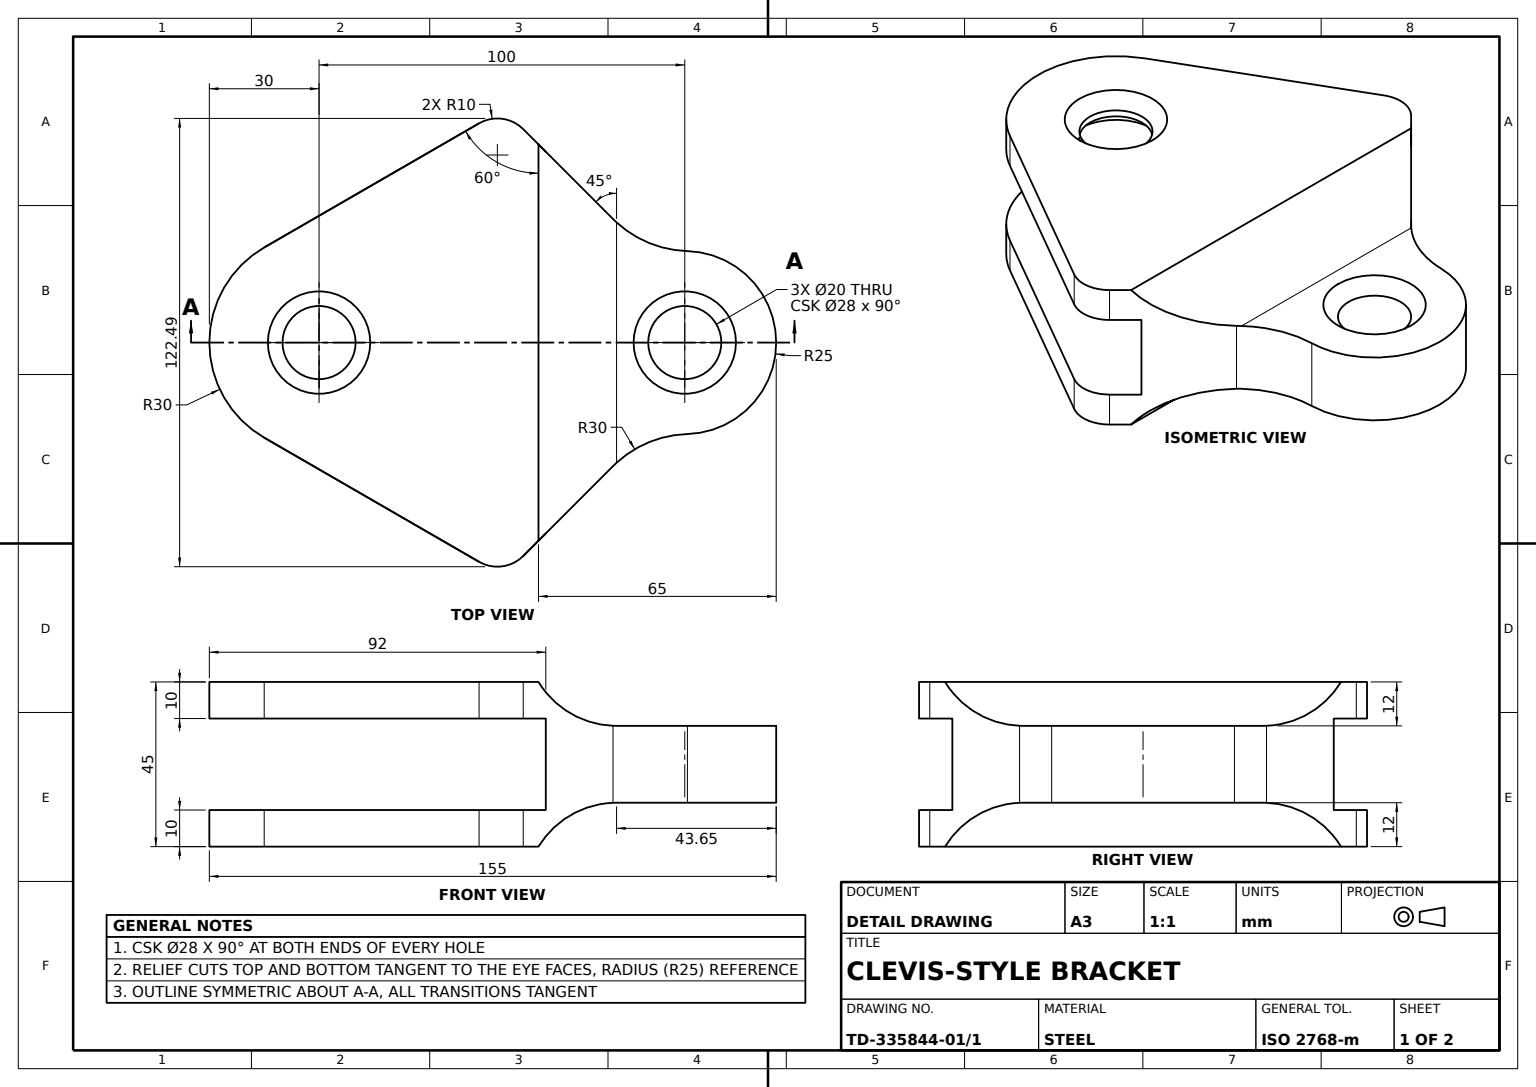
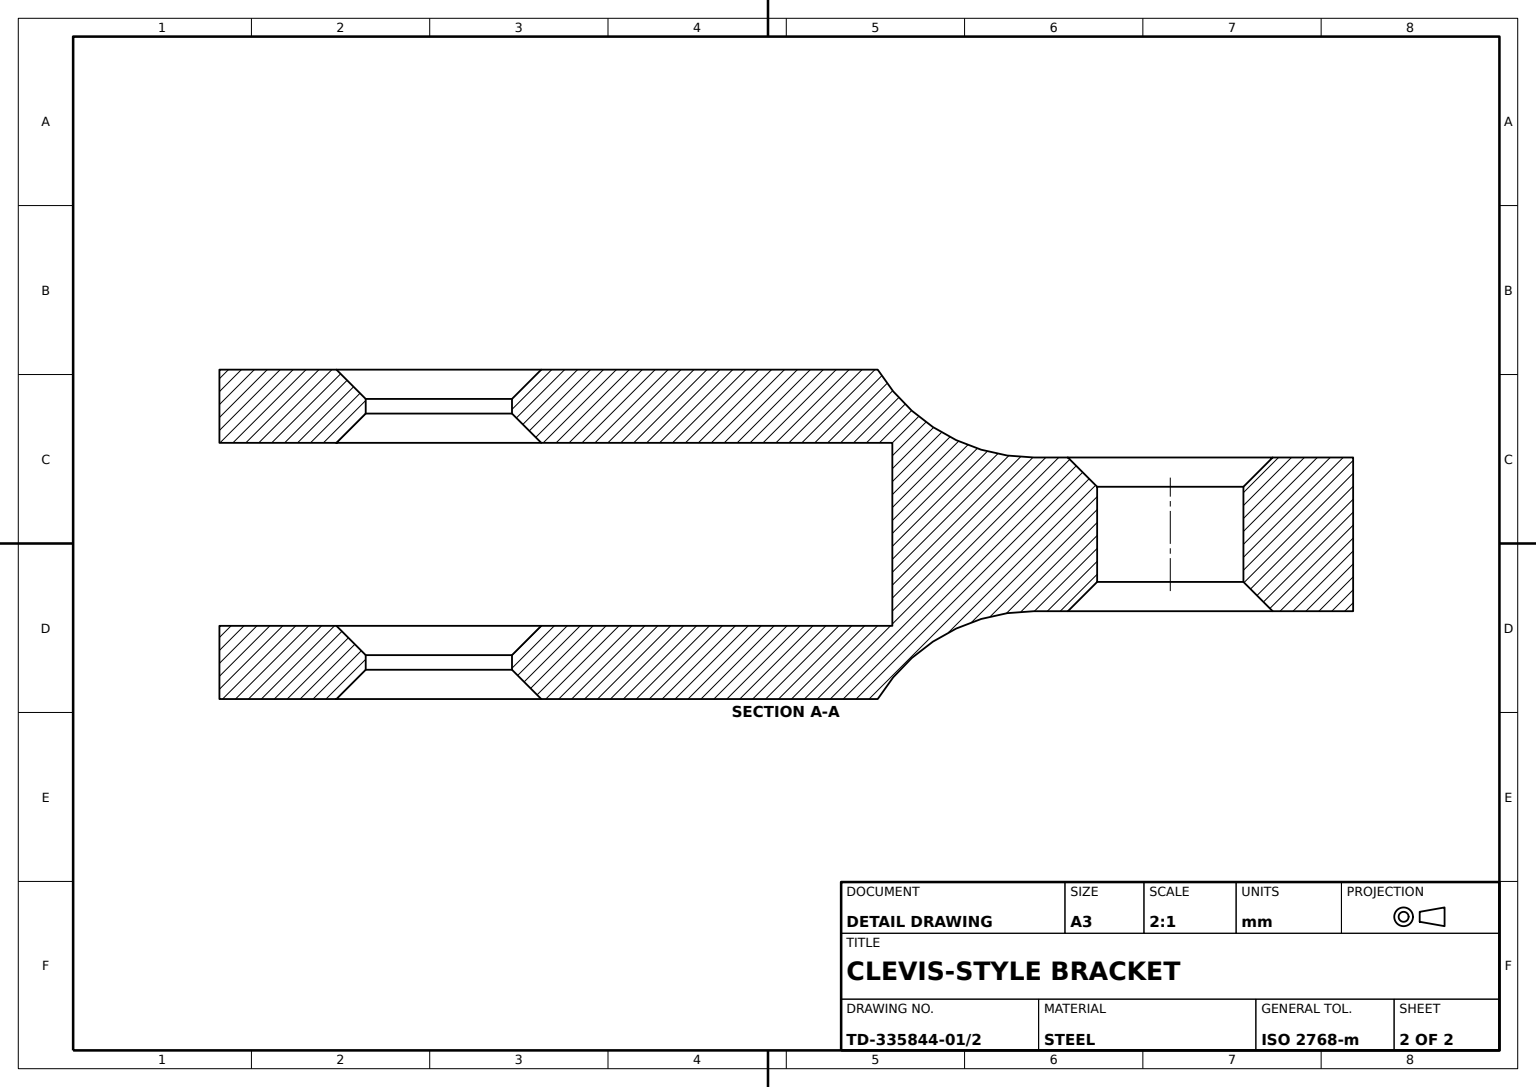
ISO-10303-21;
HEADER;
FILE_DESCRIPTION((''),'2;1');
FILE_NAME('','',(''),(''),'','','');
FILE_SCHEMA(('AUTOMOTIVE_DESIGN'));
ENDSEC;
DATA;
#1=APPLICATION_CONTEXT('');
#2=PRODUCT_CONTEXT('',#1,'mechanical');
#3=PRODUCT('','','',(#2));
#4=PRODUCT_DEFINITION_FORMATION('','',#3);
#5=PRODUCT_DEFINITION_CONTEXT('',#1,'design');
#6=PRODUCT_DEFINITION('','',#4,#5);
#7=PRODUCT_DEFINITION_SHAPE('','',#6);
#8=(LENGTH_UNIT()NAMED_UNIT(*)SI_UNIT(.MILLI.,.METRE.));
#9=(NAMED_UNIT(*)PLANE_ANGLE_UNIT()SI_UNIT($,.RADIAN.));
#10=(NAMED_UNIT(*)SI_UNIT($,.STERADIAN.)SOLID_ANGLE_UNIT());
#11=UNCERTAINTY_MEASURE_WITH_UNIT(LENGTH_MEASURE(1.E-05),#8,'distance_accuracy_value','');
#12=(GEOMETRIC_REPRESENTATION_CONTEXT(3)GLOBAL_UNCERTAINTY_ASSIGNED_CONTEXT((#11))GLOBAL_UNIT_ASSIGNED_CONTEXT((#8,#9,#10))REPRESENTATION_CONTEXT('',''));
#13=CARTESIAN_POINT('',(0.,-10.5,-86.));
#14=VERTEX_POINT('',#13);
#15=CARTESIAN_POINT('',(0.,-10.5,-114.));
#16=VERTEX_POINT('',#15);
#17=CARTESIAN_POINT('',(0.,-10.5,-100.));
#18=DIRECTION('',(0.,1.,0.));
#19=DIRECTION('',(0.,0.,1.));
#20=AXIS2_PLACEMENT_3D('',#17,#18,#19);
#21=CIRCLE('',#20,14.);
#22=EDGE_CURVE('',#14,#16,#21,.T.);
#23=ORIENTED_EDGE('',*,*,#22,.F.);
#24=CARTESIAN_POINT('',(0.,-6.5,-90.));
#25=VERTEX_POINT('',#24);
#26=DIRECTION('',(0.,-0.707106781,0.707106781));
#27=VECTOR('',#26,1000.);
#28=LINE('',#13,#27);
#29=EDGE_CURVE('',#25,#14,#28,.T.);
#30=ORIENTED_EDGE('',*,*,#29,.F.);
#31=CARTESIAN_POINT('',(0.,-6.5,-110.));
#32=VERTEX_POINT('',#31);
#33=CARTESIAN_POINT('',(0.,-6.5,-100.));
#34=DIRECTION('',(0.,-1.,0.));
#35=AXIS2_PLACEMENT_3D('',#33,#34,#19);
#36=CIRCLE('',#35,10.);
#37=EDGE_CURVE('',#32,#25,#36,.T.);
#38=ORIENTED_EDGE('',*,*,#37,.F.);
#39=DIRECTION('',(0.,-0.707106781,-0.707106781));
#40=VECTOR('',#39,1000.);
#41=LINE('',#15,#40);
#42=EDGE_CURVE('',#32,#16,#41,.T.);
#43=ORIENTED_EDGE('',*,*,#42,.T.);
#44=EDGE_LOOP('',(#23,#30,#38,#43));
#45=FACE_OUTER_BOUND('',#44,.T.);
#46=DIRECTION('',(0.,0.,-1.));
#47=AXIS2_PLACEMENT_3D('',#17,#34,#46);
#48=CONICAL_SURFACE('',#47,14.,0.785398163);
#49=ADVANCED_FACE('',(#45),#48,.F.);
#50=CARTESIAN_POINT('',(0.,16.5,-10.));
#51=VERTEX_POINT('',#50);
#52=CARTESIAN_POINT('',(0.,16.5,10.));
#53=VERTEX_POINT('',#52);
#54=CARTESIAN_POINT('',(0.,16.5,0.));
#55=AXIS2_PLACEMENT_3D('',#54,#34,#19);
#56=CIRCLE('',#55,10.);
#57=EDGE_CURVE('',#51,#53,#56,.T.);
#58=ORIENTED_EDGE('',*,*,#57,.F.);
#59=CARTESIAN_POINT('',(0.,12.5,-14.));
#60=VERTEX_POINT('',#59);
#61=LINE('',#59,#40);
#62=EDGE_CURVE('',#51,#60,#61,.T.);
#63=ORIENTED_EDGE('',*,*,#62,.T.);
#64=CARTESIAN_POINT('',(0.,12.5,14.));
#65=VERTEX_POINT('',#64);
#66=CARTESIAN_POINT('',(0.,12.5,0.));
#67=AXIS2_PLACEMENT_3D('',#66,#18,#19);
#68=CIRCLE('',#67,14.);
#69=EDGE_CURVE('',#65,#60,#68,.T.);
#70=ORIENTED_EDGE('',*,*,#69,.F.);
#71=LINE('',#64,#27);
#72=EDGE_CURVE('',#53,#65,#71,.T.);
#73=ORIENTED_EDGE('',*,*,#72,.F.);
#74=EDGE_LOOP('',(#58,#63,#70,#73));
#75=FACE_OUTER_BOUND('',#74,.T.);
#76=AXIS2_PLACEMENT_3D('',#66,#34,#46);
#77=CONICAL_SURFACE('',#76,14.,0.785398163);
#78=ADVANCED_FACE('',(#75),#77,.F.);
#79=CARTESIAN_POINT('',(25.980762,-12.5,15.));
#80=VERTEX_POINT('',#79);
#81=CARTESIAN_POINT('',(-25.980762,-12.5,15.));
#82=VERTEX_POINT('',#81);
#83=CARTESIAN_POINT('',(0.,-12.5,0.));
#84=AXIS2_PLACEMENT_3D('',#83,#34,#46);
#85=CIRCLE('',#84,30.);
#86=EDGE_CURVE('',#80,#82,#85,.T.);
#87=ORIENTED_EDGE('',*,*,#86,.T.);
#88=CARTESIAN_POINT('',(-25.980762,-22.5,15.));
#89=VERTEX_POINT('',#88);
#90=CARTESIAN_POINT('',(-25.980762,22.5,15.));
#91=VECTOR('',#34,1000.);
#92=LINE('',#90,#91);
#93=EDGE_CURVE('',#82,#89,#92,.T.);
#94=ORIENTED_EDGE('',*,*,#93,.T.);
#95=CARTESIAN_POINT('',(25.980762,-22.5,15.));
#96=VERTEX_POINT('',#95);
#97=CARTESIAN_POINT('',(0.,-22.5,0.));
#98=AXIS2_PLACEMENT_3D('',#97,#18,#19);
#99=CIRCLE('',#98,30.);
#100=EDGE_CURVE('',#89,#96,#99,.T.);
#101=ORIENTED_EDGE('',*,*,#100,.T.);
#102=CARTESIAN_POINT('',(25.980762,22.5,15.));
#103=LINE('',#102,#91);
#104=EDGE_CURVE('',#80,#96,#103,.T.);
#105=ORIENTED_EDGE('',*,*,#104,.F.);
#106=EDGE_LOOP('',(#87,#94,#101,#105));
#107=FACE_OUTER_BOUND('',#106,.T.);
#108=CARTESIAN_POINT('',(0.,22.5,0.));
#109=AXIS2_PLACEMENT_3D('',#108,#34,#46);
#110=CYLINDRICAL_SURFACE('',#109,30.);
#111=ADVANCED_FACE('',(#107),#110,.T.);
#112=CARTESIAN_POINT('',(0.,-16.5,-10.));
#113=VERTEX_POINT('',#112);
#114=CARTESIAN_POINT('',(0.,-16.5,10.));
#115=VERTEX_POINT('',#114);
#116=CARTESIAN_POINT('',(0.,-16.5,0.));
#117=AXIS2_PLACEMENT_3D('',#116,#18,#46);
#118=CIRCLE('',#117,10.);
#119=EDGE_CURVE('',#113,#115,#118,.T.);
#120=ORIENTED_EDGE('',*,*,#119,.F.);
#121=CARTESIAN_POINT('',(0.,-12.5,-14.));
#122=VERTEX_POINT('',#121);
#123=DIRECTION('',(0.,0.707106781,-0.707106781));
#124=VECTOR('',#123,1000.);
#125=LINE('',#121,#124);
#126=EDGE_CURVE('',#113,#122,#125,.T.);
#127=ORIENTED_EDGE('',*,*,#126,.T.);
#128=CARTESIAN_POINT('',(0.,-12.5,14.));
#129=VERTEX_POINT('',#128);
#130=CIRCLE('',#84,14.);
#131=EDGE_CURVE('',#129,#122,#130,.T.);
#132=ORIENTED_EDGE('',*,*,#131,.F.);
#133=DIRECTION('',(0.,0.707106781,0.707106781));
#134=VECTOR('',#133,1000.);
#135=LINE('',#128,#134);
#136=EDGE_CURVE('',#115,#129,#135,.T.);
#137=ORIENTED_EDGE('',*,*,#136,.F.);
#138=EDGE_LOOP('',(#120,#127,#132,#137));
#139=FACE_OUTER_BOUND('',#138,.T.);
#140=AXIS2_PLACEMENT_3D('',#83,#18,#19);
#141=CONICAL_SURFACE('',#140,14.,0.785398163);
#142=ADVANCED_FACE('',(#139),#141,.F.);
#143=CARTESIAN_POINT('',(33.763763,10.51905,-80.378372));
#144=VERTEX_POINT('',#143);
#145=CARTESIAN_POINT('',(54.142136,22.5,-60.));
#146=VERTEX_POINT('',#145);
#147=CARTESIAN_POINT('',(42.314948,10.853069,-71.827187));
#148=CARTESIAN_POINT('',(49.692129,15.190296,-64.450007));
#149=(BOUNDED_CURVE()B_SPLINE_CURVE(3,(#143,#147,#148,#145),.UNSPECIFIED.,.F.,.T.)B_SPLINE_CURVE_WITH_KNOTS((4,4),(4.75143027,5.736334356),.UNSPECIFIED.)CURVE()GEOMETRIC_REPRESENTATION_ITEM()RATIONAL_B_SPLINE_CURVE((1.,0.920784142,0.920784142,1.))REPRESENTATION_ITEM(''));
#150=EDGE_CURVE('',#144,#146,#149,.T.);
#151=ORIENTED_EDGE('',*,*,#150,.F.);
#152=CARTESIAN_POINT('',(32.830932,10.5,-81.354157));
#153=VERTEX_POINT('',#152);
#154=CARTESIAN_POINT('',(33.134616,10.5,-81.021831));
#155=CARTESIAN_POINT('',(33.44556,10.506621,-80.696575));
#156=B_SPLINE_CURVE_WITH_KNOTS('',3,(#152,#154,#155,#143),.UNSPECIFIED.,.F.,.F.,(4,4),(0.,0.001350071),.UNSPECIFIED.);
#157=EDGE_CURVE('',#153,#144,#156,.T.);
#158=ORIENTED_EDGE('',*,*,#157,.F.);
#159=CARTESIAN_POINT('',(-32.830932,10.5,-81.354157));
#160=VERTEX_POINT('',#159);
#161=CARTESIAN_POINT('',(-275.,10.5,-81.354157));
#162=DIRECTION('',(1.,0.,0.));
#163=VECTOR('',#162,1000.);
#164=LINE('',#161,#163);
#165=EDGE_CURVE('',#160,#153,#164,.T.);
#166=ORIENTED_EDGE('',*,*,#165,.F.);
#167=CARTESIAN_POINT('',(-33.763763,10.51905,-80.378372));
#168=VERTEX_POINT('',#167);
#169=CARTESIAN_POINT('',(-33.44556,10.506621,-80.696575));
#170=CARTESIAN_POINT('',(-33.134616,10.5,-81.021831));
#171=B_SPLINE_CURVE_WITH_KNOTS('',3,(#167,#169,#170,#159),.UNSPECIFIED.,.F.,.F.,(4,4),(0.,0.001350071),.UNSPECIFIED.);
#172=EDGE_CURVE('',#168,#160,#171,.T.);
#173=ORIENTED_EDGE('',*,*,#172,.F.);
#174=CARTESIAN_POINT('',(-54.142136,22.5,-60.));
#175=VERTEX_POINT('',#174);
#176=CARTESIAN_POINT('',(-49.692129,15.190296,-64.450007));
#177=CARTESIAN_POINT('',(-42.314948,10.853069,-71.827187));
#178=(BOUNDED_CURVE()B_SPLINE_CURVE(3,(#174,#176,#177,#167),.UNSPECIFIED.,.F.,.T.)B_SPLINE_CURVE_WITH_KNOTS((4,4),(3.688443604,4.67334769),.UNSPECIFIED.)CURVE()GEOMETRIC_REPRESENTATION_ITEM()RATIONAL_B_SPLINE_CURVE((1.,0.920784142,0.920784142,1.))REPRESENTATION_ITEM(''));
#179=EDGE_CURVE('',#175,#168,#178,.T.);
#180=ORIENTED_EDGE('',*,*,#179,.F.);
#181=CARTESIAN_POINT('',(-275.,22.5,-60.));
#182=LINE('',#181,#163);
#183=EDGE_CURVE('',#175,#146,#182,.T.);
#184=ORIENTED_EDGE('',*,*,#183,.T.);
#185=EDGE_LOOP('',(#151,#158,#166,#173,#180,#184));
#186=FACE_OUTER_BOUND('',#185,.T.);
#187=CARTESIAN_POINT('',(-275.,35.5,-81.354157));
#188=AXIS2_PLACEMENT_3D('',#187,#162,#46);
#189=CYLINDRICAL_SURFACE('',#188,25.);
#190=ADVANCED_FACE('',(#186),#189,.F.);
#191=VERTEX_POINT('',#102);
#192=CARTESIAN_POINT('',(25.980762,12.5,15.));
#193=VERTEX_POINT('',#192);
#194=EDGE_CURVE('',#191,#193,#103,.T.);
#195=ORIENTED_EDGE('',*,*,#194,.T.);
#196=CARTESIAN_POINT('',(59.903811,12.5,-43.756443));
#197=VERTEX_POINT('',#196);
#198=DIRECTION('',(0.5,0.,-0.866025404));
#199=VECTOR('',#198,1000.);
#200=LINE('',#192,#199);
#201=EDGE_CURVE('',#193,#197,#200,.T.);
#202=ORIENTED_EDGE('',*,*,#201,.T.);
#203=CARTESIAN_POINT('',(59.903811,22.5,-43.756443));
#204=VERTEX_POINT('',#203);
#205=LINE('',#203,#91);
#206=EDGE_CURVE('',#204,#197,#205,.T.);
#207=ORIENTED_EDGE('',*,*,#206,.F.);
#208=LINE('',#102,#199);
#209=EDGE_CURVE('',#191,#204,#208,.T.);
#210=ORIENTED_EDGE('',*,*,#209,.F.);
#211=EDGE_LOOP('',(#195,#202,#207,#210));
#212=FACE_OUTER_BOUND('',#211,.T.);
#213=DIRECTION('',(-0.866025404,0.,-0.5));
#214=DIRECTION('',(-0.5,0.,0.866025404));
#215=AXIS2_PLACEMENT_3D('',#102,#213,#214);
#216=PLANE('',#215);
#217=ADVANCED_FACE('',(#212),#216,.F.);
#218=ORIENTED_EDGE('',*,*,#172,.T.);
#219=CARTESIAN_POINT('',(-24.98953,10.5,-100.723443));
#220=VERTEX_POINT('',#219);
#221=CARTESIAN_POINT('',(-54.976967,10.5,-101.591576));
#222=AXIS2_PLACEMENT_3D('',#221,#18,#46);
#223=CIRCLE('',#222,30.);
#224=EDGE_CURVE('',#160,#220,#223,.T.);
#225=ORIENTED_EDGE('',*,*,#224,.T.);
#226=CARTESIAN_POINT('',(-24.98953,-10.5,-100.723443));
#227=VERTEX_POINT('',#226);
#228=CARTESIAN_POINT('',(-24.98953,22.5,-100.723443));
#229=LINE('',#228,#91);
#230=EDGE_CURVE('',#220,#227,#229,.T.);
#231=ORIENTED_EDGE('',*,*,#230,.T.);
#232=CARTESIAN_POINT('',(-32.830932,-10.5,-81.354157));
#233=VERTEX_POINT('',#232);
#234=CARTESIAN_POINT('',(-54.976967,-10.5,-101.591576));
#235=AXIS2_PLACEMENT_3D('',#234,#34,#19);
#236=CIRCLE('',#235,30.);
#237=EDGE_CURVE('',#227,#233,#236,.T.);
#238=ORIENTED_EDGE('',*,*,#237,.T.);
#239=CARTESIAN_POINT('',(-33.763763,-10.51905,-80.378372));
#240=VERTEX_POINT('',#239);
#241=CARTESIAN_POINT('',(-33.134616,-10.5,-81.021831));
#242=CARTESIAN_POINT('',(-33.44556,-10.506621,-80.696575));
#243=B_SPLINE_CURVE_WITH_KNOTS('',3,(#232,#241,#242,#239),.UNSPECIFIED.,.F.,.F.,(4,4),(0.,0.001350071),.UNSPECIFIED.);
#244=EDGE_CURVE('',#233,#240,#243,.T.);
#245=ORIENTED_EDGE('',*,*,#244,.T.);
#246=CARTESIAN_POINT('',(-33.763763,22.5,-80.378372));
#247=LINE('',#246,#91);
#248=EDGE_CURVE('',#168,#240,#247,.T.);
#249=ORIENTED_EDGE('',*,*,#248,.F.);
#250=EDGE_LOOP('',(#218,#225,#231,#238,#245,#249));
#251=FACE_OUTER_BOUND('',#250,.T.);
#252=CARTESIAN_POINT('',(-54.976967,22.5,-101.591576));
#253=AXIS2_PLACEMENT_3D('',#252,#34,#46);
#254=CYLINDRICAL_SURFACE('',#253,30.);
#255=ADVANCED_FACE('',(#251),#254,.F.);
#256=ORIENTED_EDGE('',*,*,#126,.F.);
#257=EDGE_CURVE('',#115,#113,#118,.T.);
#258=ORIENTED_EDGE('',*,*,#257,.F.);
#259=ORIENTED_EDGE('',*,*,#136,.T.);
#260=EDGE_CURVE('',#122,#129,#130,.T.);
#261=ORIENTED_EDGE('',*,*,#260,.F.);
#262=EDGE_LOOP('',(#256,#258,#259,#261));
#263=FACE_OUTER_BOUND('',#262,.T.);
#264=ADVANCED_FACE('',(#263),#141,.F.);
#265=CARTESIAN_POINT('',(-52.142136,-12.5,-62.));
#266=VERTEX_POINT('',#265);
#267=CARTESIAN_POINT('',(52.142136,-12.5,-62.));
#268=VERTEX_POINT('',#267);
#269=CARTESIAN_POINT('',(-275.,-12.5,-62.));
#270=LINE('',#269,#163);
#271=EDGE_CURVE('',#266,#268,#270,.T.);
#272=ORIENTED_EDGE('',*,*,#271,.T.);
#273=CARTESIAN_POINT('',(52.142136,12.5,-62.));
#274=VERTEX_POINT('',#273);
#275=CARTESIAN_POINT('',(52.142136,22.5,-62.));
#276=LINE('',#275,#91);
#277=EDGE_CURVE('',#274,#268,#276,.T.);
#278=ORIENTED_EDGE('',*,*,#277,.F.);
#279=CARTESIAN_POINT('',(-52.142136,12.5,-62.));
#280=VERTEX_POINT('',#279);
#281=CARTESIAN_POINT('',(-275.,12.5,-62.));
#282=LINE('',#281,#163);
#283=EDGE_CURVE('',#280,#274,#282,.T.);
#284=ORIENTED_EDGE('',*,*,#283,.F.);
#285=CARTESIAN_POINT('',(-52.142136,22.5,-62.));
#286=VECTOR('',#18,1000.);
#287=LINE('',#285,#286);
#288=EDGE_CURVE('',#266,#280,#287,.T.);
#289=ORIENTED_EDGE('',*,*,#288,.F.);
#290=EDGE_LOOP('',(#272,#278,#284,#289));
#291=FACE_OUTER_BOUND('',#290,.T.);
#292=DIRECTION('',(-1.,0.,0.));
#293=AXIS2_PLACEMENT_3D('',#281,#46,#292);
#294=PLANE('',#293);
#295=ADVANCED_FACE('',(#291),#294,.F.);
#296=CARTESIAN_POINT('',(0.,-22.5,14.));
#297=VERTEX_POINT('',#296);
#298=CARTESIAN_POINT('',(0.,-22.5,-14.));
#299=VERTEX_POINT('',#298);
#300=AXIS2_PLACEMENT_3D('',#97,#18,#46);
#301=CIRCLE('',#300,14.);
#302=EDGE_CURVE('',#297,#299,#301,.T.);
#303=ORIENTED_EDGE('',*,*,#302,.F.);
#304=CARTESIAN_POINT('',(0.,-18.5,10.));
#305=VERTEX_POINT('',#304);
#306=LINE('',#296,#27);
#307=EDGE_CURVE('',#305,#297,#306,.T.);
#308=ORIENTED_EDGE('',*,*,#307,.F.);
#309=CARTESIAN_POINT('',(0.,-18.5,-10.));
#310=VERTEX_POINT('',#309);
#311=CARTESIAN_POINT('',(0.,-18.5,0.));
#312=AXIS2_PLACEMENT_3D('',#311,#34,#46);
#313=CIRCLE('',#312,10.);
#314=EDGE_CURVE('',#310,#305,#313,.T.);
#315=ORIENTED_EDGE('',*,*,#314,.F.);
#316=LINE('',#298,#40);
#317=EDGE_CURVE('',#310,#299,#316,.T.);
#318=ORIENTED_EDGE('',*,*,#317,.T.);
#319=EDGE_LOOP('',(#303,#308,#315,#318));
#320=FACE_OUTER_BOUND('',#319,.T.);
#321=AXIS2_PLACEMENT_3D('',#97,#34,#46);
#322=CONICAL_SURFACE('',#321,14.,0.785398163);
#323=ADVANCED_FACE('',(#320),#322,.F.);
#324=ORIENTED_EDGE('',*,*,#93,.F.);
#325=CARTESIAN_POINT('',(-59.903811,-12.5,-43.756443));
#326=VERTEX_POINT('',#325);
#327=DIRECTION('',(-0.5,0.,-0.866025404));
#328=VECTOR('',#327,1000.);
#329=LINE('',#81,#328);
#330=EDGE_CURVE('',#82,#326,#329,.T.);
#331=ORIENTED_EDGE('',*,*,#330,.T.);
#332=CARTESIAN_POINT('',(-59.903811,-22.5,-43.756443));
#333=VERTEX_POINT('',#332);
#334=CARTESIAN_POINT('',(-59.903811,22.5,-43.756443));
#335=LINE('',#334,#91);
#336=EDGE_CURVE('',#326,#333,#335,.T.);
#337=ORIENTED_EDGE('',*,*,#336,.T.);
#338=DIRECTION('',(0.5,0.,0.866025404));
#339=VECTOR('',#338,1000.);
#340=LINE('',#88,#339);
#341=EDGE_CURVE('',#333,#89,#340,.T.);
#342=ORIENTED_EDGE('',*,*,#341,.T.);
#343=EDGE_LOOP('',(#324,#331,#337,#342));
#344=FACE_OUTER_BOUND('',#343,.T.);
#345=DIRECTION('',(0.866025404,0.,-0.5));
#346=AXIS2_PLACEMENT_3D('',#90,#345,#327);
#347=PLANE('',#346);
#348=ADVANCED_FACE('',(#344),#347,.F.);
#349=CARTESIAN_POINT('',(58.314624,-12.5,-55.827511));
#350=VERTEX_POINT('',#349);
#351=CARTESIAN_POINT('',(59.903811,-12.5,-43.756443));
#352=VERTEX_POINT('',#351);
#353=CARTESIAN_POINT('',(51.243557,-12.5,-48.756443));
#354=AXIS2_PLACEMENT_3D('',#353,#34,#46);
#355=CIRCLE('',#354,10.);
#356=EDGE_CURVE('',#350,#352,#355,.T.);
#357=ORIENTED_EDGE('',*,*,#356,.T.);
#358=CARTESIAN_POINT('',(59.903811,-22.5,-43.756443));
#359=VERTEX_POINT('',#358);
#360=EDGE_CURVE('',#352,#359,#205,.T.);
#361=ORIENTED_EDGE('',*,*,#360,.T.);
#362=CARTESIAN_POINT('',(58.314624,-22.5,-55.827511));
#363=VERTEX_POINT('',#362);
#364=CARTESIAN_POINT('',(51.243557,-22.5,-48.756443));
#365=AXIS2_PLACEMENT_3D('',#364,#18,#46);
#366=CIRCLE('',#365,10.);
#367=EDGE_CURVE('',#359,#363,#366,.T.);
#368=ORIENTED_EDGE('',*,*,#367,.T.);
#369=CARTESIAN_POINT('',(58.314624,22.5,-55.827511));
#370=LINE('',#369,#91);
#371=EDGE_CURVE('',#350,#363,#370,.T.);
#372=ORIENTED_EDGE('',*,*,#371,.F.);
#373=EDGE_LOOP('',(#357,#361,#368,#372));
#374=FACE_OUTER_BOUND('',#373,.T.);
#375=CARTESIAN_POINT('',(51.243557,22.5,-48.756443));
#376=AXIS2_PLACEMENT_3D('',#375,#34,#46);
#377=CYLINDRICAL_SURFACE('',#376,10.);
#378=ADVANCED_FACE('',(#374),#377,.T.);
#379=CARTESIAN_POINT('',(32.830932,-10.5,-81.354157));
#380=VERTEX_POINT('',#379);
#381=CARTESIAN_POINT('',(24.98953,-10.5,-100.723443));
#382=VERTEX_POINT('',#381);
#383=CARTESIAN_POINT('',(54.976967,-10.5,-101.591576));
#384=AXIS2_PLACEMENT_3D('',#383,#34,#19);
#385=CIRCLE('',#384,30.);
#386=EDGE_CURVE('',#380,#382,#385,.T.);
#387=ORIENTED_EDGE('',*,*,#386,.T.);
#388=CARTESIAN_POINT('',(24.98953,10.5,-100.723443));
#389=VERTEX_POINT('',#388);
#390=CARTESIAN_POINT('',(24.98953,22.5,-100.723443));
#391=LINE('',#390,#91);
#392=EDGE_CURVE('',#389,#382,#391,.T.);
#393=ORIENTED_EDGE('',*,*,#392,.F.);
#394=CARTESIAN_POINT('',(54.976967,10.5,-101.591576));
#395=AXIS2_PLACEMENT_3D('',#394,#18,#46);
#396=CIRCLE('',#395,30.);
#397=EDGE_CURVE('',#389,#153,#396,.T.);
#398=ORIENTED_EDGE('',*,*,#397,.T.);
#399=ORIENTED_EDGE('',*,*,#157,.T.);
#400=CARTESIAN_POINT('',(33.763763,-10.51905,-80.378372));
#401=VERTEX_POINT('',#400);
#402=CARTESIAN_POINT('',(33.763763,22.5,-80.378372));
#403=LINE('',#402,#91);
#404=EDGE_CURVE('',#144,#401,#403,.T.);
#405=ORIENTED_EDGE('',*,*,#404,.T.);
#406=CARTESIAN_POINT('',(33.44556,-10.506621,-80.696575));
#407=CARTESIAN_POINT('',(33.134616,-10.5,-81.021831));
#408=B_SPLINE_CURVE_WITH_KNOTS('',3,(#400,#406,#407,#379),.UNSPECIFIED.,.F.,.F.,(4,4),(0.,0.001350071),.UNSPECIFIED.);
#409=EDGE_CURVE('',#401,#380,#408,.T.);
#410=ORIENTED_EDGE('',*,*,#409,.T.);
#411=EDGE_LOOP('',(#387,#393,#398,#399,#405,#410));
#412=FACE_OUTER_BOUND('',#411,.T.);
#413=CARTESIAN_POINT('',(54.976967,22.5,-101.591576));
#414=AXIS2_PLACEMENT_3D('',#413,#34,#46);
#415=CYLINDRICAL_SURFACE('',#414,30.);
#416=ADVANCED_FACE('',(#412),#415,.F.);
#417=CARTESIAN_POINT('',(-58.314624,22.5,-55.827511));
#418=VERTEX_POINT('',#417);
#419=CARTESIAN_POINT('',(-58.314624,12.5,-55.827511));
#420=VERTEX_POINT('',#419);
#421=LINE('',#417,#91);
#422=EDGE_CURVE('',#418,#420,#421,.T.);
#423=ORIENTED_EDGE('',*,*,#422,.F.);
#424=DIRECTION('',(-0.707106781,0.,0.707106781));
#425=VECTOR('',#424,1000.);
#426=LINE('',#246,#425);
#427=EDGE_CURVE('',#175,#418,#426,.T.);
#428=ORIENTED_EDGE('',*,*,#427,.F.);
#429=ORIENTED_EDGE('',*,*,#179,.T.);
#430=ORIENTED_EDGE('',*,*,#248,.T.);
#431=CARTESIAN_POINT('',(-54.142136,-22.5,-60.));
#432=VERTEX_POINT('',#431);
#433=CARTESIAN_POINT('',(-42.314948,-10.853069,-71.827187));
#434=CARTESIAN_POINT('',(-49.692129,-15.190296,-64.450007));
#435=(BOUNDED_CURVE()B_SPLINE_CURVE(3,(#239,#433,#434,#431),.UNSPECIFIED.,.F.,.T.)B_SPLINE_CURVE_WITH_KNOTS((4,4),(1.609837617,2.594741703),.UNSPECIFIED.)CURVE()GEOMETRIC_REPRESENTATION_ITEM()RATIONAL_B_SPLINE_CURVE((1.,0.920784142,0.920784142,1.))REPRESENTATION_ITEM(''));
#436=EDGE_CURVE('',#240,#432,#435,.T.);
#437=ORIENTED_EDGE('',*,*,#436,.T.);
#438=CARTESIAN_POINT('',(-58.314624,-22.5,-55.827511));
#439=VERTEX_POINT('',#438);
#440=CARTESIAN_POINT('',(-33.763763,-22.5,-80.378372));
#441=LINE('',#440,#425);
#442=EDGE_CURVE('',#432,#439,#441,.T.);
#443=ORIENTED_EDGE('',*,*,#442,.T.);
#444=CARTESIAN_POINT('',(-58.314624,-12.5,-55.827511));
#445=VERTEX_POINT('',#444);
#446=EDGE_CURVE('',#445,#439,#421,.T.);
#447=ORIENTED_EDGE('',*,*,#446,.F.);
#448=CARTESIAN_POINT('',(-33.763763,-12.5,-80.378372));
#449=DIRECTION('',(0.707106781,0.,-0.707106781));
#450=VECTOR('',#449,1000.);
#451=LINE('',#448,#450);
#452=EDGE_CURVE('',#445,#266,#451,.T.);
#453=ORIENTED_EDGE('',*,*,#452,.T.);
#454=ORIENTED_EDGE('',*,*,#288,.T.);
#455=CARTESIAN_POINT('',(-33.763763,12.5,-80.378372));
#456=LINE('',#455,#425);
#457=EDGE_CURVE('',#280,#420,#456,.T.);
#458=ORIENTED_EDGE('',*,*,#457,.T.);
#459=EDGE_LOOP('',(#423,#428,#429,#430,#437,#443,#447,#453,#454,#458));
#460=FACE_OUTER_BOUND('',#459,.T.);
#461=DIRECTION('',(0.707106781,0.,0.707106781));
#462=AXIS2_PLACEMENT_3D('',#246,#461,#449);
#463=PLANE('',#462);
#464=ADVANCED_FACE('',(#460),#463,.F.);
#465=ORIENTED_EDGE('',*,*,#356,.F.);
#466=CARTESIAN_POINT('',(33.763763,-12.5,-80.378372));
#467=VECTOR('',#461,1000.);
#468=LINE('',#466,#467);
#469=EDGE_CURVE('',#268,#350,#468,.T.);
#470=ORIENTED_EDGE('',*,*,#469,.F.);
#471=ORIENTED_EDGE('',*,*,#271,.F.);
#472=ORIENTED_EDGE('',*,*,#452,.F.);
#473=CARTESIAN_POINT('',(-51.243557,-12.5,-48.756443));
#474=AXIS2_PLACEMENT_3D('',#473,#34,#46);
#475=CIRCLE('',#474,10.);
#476=EDGE_CURVE('',#326,#445,#475,.T.);
#477=ORIENTED_EDGE('',*,*,#476,.F.);
#478=ORIENTED_EDGE('',*,*,#330,.F.);
#479=ORIENTED_EDGE('',*,*,#86,.F.);
#480=VECTOR('',#214,1000.);
#481=LINE('',#79,#480);
#482=EDGE_CURVE('',#352,#80,#481,.T.);
#483=ORIENTED_EDGE('',*,*,#482,.F.);
#484=EDGE_LOOP('',(#465,#470,#471,#472,#477,#478,#479,#483));
#485=FACE_OUTER_BOUND('',#484,.T.);
#486=ORIENTED_EDGE('',*,*,#260,.T.);
#487=ORIENTED_EDGE('',*,*,#131,.T.);
#488=EDGE_LOOP('',(#486,#487));
#489=FACE_BOUND('',#488,.T.);
#490=AXIS2_PLACEMENT_3D('',#269,#34,#46);
#491=PLANE('',#490);
#492=ADVANCED_FACE('',(#485,#489),#491,.F.);
#493=CARTESIAN_POINT('',(0.,10.5,-114.));
#494=VERTEX_POINT('',#493);
#495=CARTESIAN_POINT('',(0.,10.5,-86.));
#496=VERTEX_POINT('',#495);
#497=CARTESIAN_POINT('',(0.,10.5,-100.));
#498=AXIS2_PLACEMENT_3D('',#497,#34,#46);
#499=CIRCLE('',#498,14.);
#500=EDGE_CURVE('',#494,#496,#499,.T.);
#501=ORIENTED_EDGE('',*,*,#500,.F.);
#502=CARTESIAN_POINT('',(0.,6.5,-110.));
#503=VERTEX_POINT('',#502);
#504=LINE('',#493,#124);
#505=EDGE_CURVE('',#503,#494,#504,.T.);
#506=ORIENTED_EDGE('',*,*,#505,.F.);
#507=CARTESIAN_POINT('',(0.,6.5,-90.));
#508=VERTEX_POINT('',#507);
#509=CARTESIAN_POINT('',(0.,6.5,-100.));
#510=AXIS2_PLACEMENT_3D('',#509,#18,#46);
#511=CIRCLE('',#510,10.);
#512=EDGE_CURVE('',#508,#503,#511,.T.);
#513=ORIENTED_EDGE('',*,*,#512,.F.);
#514=LINE('',#495,#134);
#515=EDGE_CURVE('',#508,#496,#514,.T.);
#516=ORIENTED_EDGE('',*,*,#515,.T.);
#517=EDGE_LOOP('',(#501,#506,#513,#516));
#518=FACE_OUTER_BOUND('',#517,.T.);
#519=AXIS2_PLACEMENT_3D('',#497,#18,#19);
#520=CONICAL_SURFACE('',#519,14.,0.785398163);
#521=ADVANCED_FACE('',(#518),#520,.F.);
#522=ORIENTED_EDGE('',*,*,#500,.T.);
#523=EDGE_CURVE('',#496,#494,#499,.T.);
#524=ORIENTED_EDGE('',*,*,#523,.T.);
#525=EDGE_LOOP('',(#522,#524));
#526=FACE_BOUND('',#525,.T.);
#527=ORIENTED_EDGE('',*,*,#165,.T.);
#528=ORIENTED_EDGE('',*,*,#397,.F.);
#529=CARTESIAN_POINT('',(0.,10.5,-125.));
#530=VERTEX_POINT('',#529);
#531=CIRCLE('',#498,25.);
#532=EDGE_CURVE('',#530,#389,#531,.T.);
#533=ORIENTED_EDGE('',*,*,#532,.F.);
#534=EDGE_CURVE('',#220,#530,#531,.T.);
#535=ORIENTED_EDGE('',*,*,#534,.F.);
#536=ORIENTED_EDGE('',*,*,#224,.F.);
#537=EDGE_LOOP('',(#527,#528,#533,#535,#536));
#538=FACE_OUTER_BOUND('',#537,.T.);
#539=CARTESIAN_POINT('',(-275.,10.5,-125.));
#540=AXIS2_PLACEMENT_3D('',#539,#34,#46);
#541=PLANE('',#540);
#542=ADVANCED_FACE('',(#526,#538),#541,.F.);
#543=ORIENTED_EDGE('',*,*,#206,.T.);
#544=CARTESIAN_POINT('',(58.314624,12.5,-55.827511));
#545=VERTEX_POINT('',#544);
#546=CARTESIAN_POINT('',(51.243557,12.5,-48.756443));
#547=AXIS2_PLACEMENT_3D('',#546,#18,#19);
#548=CIRCLE('',#547,10.);
#549=EDGE_CURVE('',#197,#545,#548,.T.);
#550=ORIENTED_EDGE('',*,*,#549,.T.);
#551=VERTEX_POINT('',#369);
#552=EDGE_CURVE('',#551,#545,#370,.T.);
#553=ORIENTED_EDGE('',*,*,#552,.F.);
#554=AXIS2_PLACEMENT_3D('',#375,#18,#46);
#555=CIRCLE('',#554,10.);
#556=EDGE_CURVE('',#204,#551,#555,.T.);
#557=ORIENTED_EDGE('',*,*,#556,.F.);
#558=EDGE_LOOP('',(#543,#550,#553,#557));
#559=FACE_OUTER_BOUND('',#558,.T.);
#560=ADVANCED_FACE('',(#559),#377,.T.);
#561=CARTESIAN_POINT('',(0.,18.5,10.));
#562=VERTEX_POINT('',#561);
#563=CARTESIAN_POINT('',(0.,18.5,-10.));
#564=VERTEX_POINT('',#563);
#565=CARTESIAN_POINT('',(0.,18.5,0.));
#566=AXIS2_PLACEMENT_3D('',#565,#18,#46);
#567=CIRCLE('',#566,10.);
#568=EDGE_CURVE('',#562,#564,#567,.T.);
#569=ORIENTED_EDGE('',*,*,#568,.T.);
#570=CARTESIAN_POINT('',(0.,22.5,-10.));
#571=LINE('',#570,#91);
#572=EDGE_CURVE('',#564,#51,#571,.T.);
#573=ORIENTED_EDGE('',*,*,#572,.T.);
#574=ORIENTED_EDGE('',*,*,#57,.T.);
#575=CARTESIAN_POINT('',(0.,22.5,10.));
#576=LINE('',#575,#91);
#577=EDGE_CURVE('',#562,#53,#576,.T.);
#578=ORIENTED_EDGE('',*,*,#577,.F.);
#579=EDGE_LOOP('',(#569,#573,#574,#578));
#580=FACE_OUTER_BOUND('',#579,.T.);
#581=CYLINDRICAL_SURFACE('',#109,10.);
#582=ADVANCED_FACE('',(#580),#581,.F.);
#583=ORIENTED_EDGE('',*,*,#119,.T.);
#584=EDGE_CURVE('',#115,#305,#576,.T.);
#585=ORIENTED_EDGE('',*,*,#584,.T.);
#586=EDGE_CURVE('',#305,#310,#313,.T.);
#587=ORIENTED_EDGE('',*,*,#586,.T.);
#588=EDGE_CURVE('',#113,#310,#571,.T.);
#589=ORIENTED_EDGE('',*,*,#588,.F.);
#590=EDGE_LOOP('',(#583,#585,#587,#589));
#591=FACE_OUTER_BOUND('',#590,.T.);
#592=ADVANCED_FACE('',(#591),#581,.F.);
#593=ORIENTED_EDGE('',*,*,#230,.F.);
#594=ORIENTED_EDGE('',*,*,#534,.T.);
#595=CARTESIAN_POINT('',(0.,-10.5,-125.));
#596=VERTEX_POINT('',#595);
#597=CARTESIAN_POINT('',(0.,22.5,-125.));
#598=LINE('',#597,#91);
#599=EDGE_CURVE('',#530,#596,#598,.T.);
#600=ORIENTED_EDGE('',*,*,#599,.T.);
#601=CIRCLE('',#20,25.);
#602=EDGE_CURVE('',#596,#227,#601,.T.);
#603=ORIENTED_EDGE('',*,*,#602,.T.);
#604=EDGE_LOOP('',(#593,#594,#600,#603));
#605=FACE_OUTER_BOUND('',#604,.T.);
#606=CARTESIAN_POINT('',(0.,22.5,-100.));
#607=AXIS2_PLACEMENT_3D('',#606,#34,#46);
#608=CYLINDRICAL_SURFACE('',#607,25.);
#609=ADVANCED_FACE('',(#605),#608,.T.);
#610=ORIENTED_EDGE('',*,*,#302,.T.);
#611=EDGE_CURVE('',#299,#297,#301,.T.);
#612=ORIENTED_EDGE('',*,*,#611,.T.);
#613=EDGE_LOOP('',(#610,#612));
#614=FACE_BOUND('',#613,.T.);
#615=ORIENTED_EDGE('',*,*,#367,.F.);
#616=LINE('',#95,#199);
#617=EDGE_CURVE('',#96,#359,#616,.T.);
#618=ORIENTED_EDGE('',*,*,#617,.F.);
#619=ORIENTED_EDGE('',*,*,#100,.F.);
#620=ORIENTED_EDGE('',*,*,#341,.F.);
#621=CARTESIAN_POINT('',(-51.243557,-22.5,-48.756443));
#622=AXIS2_PLACEMENT_3D('',#621,#18,#19);
#623=CIRCLE('',#622,10.);
#624=EDGE_CURVE('',#439,#333,#623,.T.);
#625=ORIENTED_EDGE('',*,*,#624,.F.);
#626=ORIENTED_EDGE('',*,*,#442,.F.);
#627=CARTESIAN_POINT('',(54.142136,-22.5,-60.));
#628=VERTEX_POINT('',#627);
#629=CARTESIAN_POINT('',(-275.,-22.5,-60.));
#630=LINE('',#629,#163);
#631=EDGE_CURVE('',#432,#628,#630,.T.);
#632=ORIENTED_EDGE('',*,*,#631,.T.);
#633=CARTESIAN_POINT('',(33.763763,-22.5,-80.378372));
#634=DIRECTION('',(-0.707106781,0.,-0.707106781));
#635=VECTOR('',#634,1000.);
#636=LINE('',#633,#635);
#637=EDGE_CURVE('',#363,#628,#636,.T.);
#638=ORIENTED_EDGE('',*,*,#637,.F.);
#639=EDGE_LOOP('',(#615,#618,#619,#620,#625,#626,#632,#638));
#640=FACE_OUTER_BOUND('',#639,.T.);
#641=CARTESIAN_POINT('',(54.976967,-22.5,-101.591576));
#642=AXIS2_PLACEMENT_3D('',#641,#34,#46);
#643=PLANE('',#642);
#644=ADVANCED_FACE('',(#614,#640),#643,.T.);
#645=ORIENTED_EDGE('',*,*,#237,.F.);
#646=ORIENTED_EDGE('',*,*,#602,.F.);
#647=EDGE_CURVE('',#382,#596,#601,.T.);
#648=ORIENTED_EDGE('',*,*,#647,.F.);
#649=ORIENTED_EDGE('',*,*,#386,.F.);
#650=CARTESIAN_POINT('',(-275.,-10.5,-81.354157));
#651=LINE('',#650,#163);
#652=EDGE_CURVE('',#233,#380,#651,.T.);
#653=ORIENTED_EDGE('',*,*,#652,.F.);
#654=EDGE_LOOP('',(#645,#646,#648,#649,#653));
#655=FACE_OUTER_BOUND('',#654,.T.);
#656=EDGE_CURVE('',#16,#14,#21,.T.);
#657=ORIENTED_EDGE('',*,*,#656,.T.);
#658=ORIENTED_EDGE('',*,*,#22,.T.);
#659=EDGE_LOOP('',(#657,#658));
#660=FACE_BOUND('',#659,.T.);
#661=AXIS2_PLACEMENT_3D('',#650,#18,#19);
#662=PLANE('',#661);
#663=ADVANCED_FACE('',(#655,#660),#662,.F.);
#664=ORIENTED_EDGE('',*,*,#194,.F.);
#665=VERTEX_POINT('',#90);
#666=AXIS2_PLACEMENT_3D('',#108,#18,#19);
#667=CIRCLE('',#666,30.);
#668=EDGE_CURVE('',#665,#191,#667,.T.);
#669=ORIENTED_EDGE('',*,*,#668,.F.);
#670=CARTESIAN_POINT('',(-25.980762,12.5,15.));
#671=VERTEX_POINT('',#670);
#672=EDGE_CURVE('',#665,#671,#92,.T.);
#673=ORIENTED_EDGE('',*,*,#672,.T.);
#674=CIRCLE('',#67,30.);
#675=EDGE_CURVE('',#671,#193,#674,.T.);
#676=ORIENTED_EDGE('',*,*,#675,.T.);
#677=EDGE_LOOP('',(#664,#669,#673,#676));
#678=FACE_OUTER_BOUND('',#677,.T.);
#679=ADVANCED_FACE('',(#678),#110,.T.);
#680=CARTESIAN_POINT('',(0.,22.5,-14.));
#681=VERTEX_POINT('',#680);
#682=LINE('',#563,#124);
#683=EDGE_CURVE('',#564,#681,#682,.T.);
#684=ORIENTED_EDGE('',*,*,#683,.F.);
#685=ORIENTED_EDGE('',*,*,#568,.F.);
#686=CARTESIAN_POINT('',(0.,22.5,14.));
#687=VERTEX_POINT('',#686);
#688=LINE('',#561,#134);
#689=EDGE_CURVE('',#562,#687,#688,.T.);
#690=ORIENTED_EDGE('',*,*,#689,.T.);
#691=CIRCLE('',#109,14.);
#692=EDGE_CURVE('',#681,#687,#691,.T.);
#693=ORIENTED_EDGE('',*,*,#692,.F.);
#694=EDGE_LOOP('',(#684,#685,#690,#693));
#695=FACE_OUTER_BOUND('',#694,.T.);
#696=AXIS2_PLACEMENT_3D('',#565,#18,#19);
#697=CONICAL_SURFACE('',#696,10.,0.785398163);
#698=ADVANCED_FACE('',(#695),#697,.F.);
#699=ORIENTED_EDGE('',*,*,#523,.F.);
#700=ORIENTED_EDGE('',*,*,#515,.F.);
#701=EDGE_CURVE('',#503,#508,#511,.T.);
#702=ORIENTED_EDGE('',*,*,#701,.F.);
#703=ORIENTED_EDGE('',*,*,#505,.T.);
#704=EDGE_LOOP('',(#699,#700,#702,#703));
#705=FACE_OUTER_BOUND('',#704,.T.);
#706=ADVANCED_FACE('',(#705),#520,.F.);
#707=CARTESIAN_POINT('',(33.763763,12.5,-80.378372));
#708=LINE('',#707,#635);
#709=EDGE_CURVE('',#545,#274,#708,.T.);
#710=ORIENTED_EDGE('',*,*,#709,.F.);
#711=ORIENTED_EDGE('',*,*,#549,.F.);
#712=ORIENTED_EDGE('',*,*,#201,.F.);
#713=ORIENTED_EDGE('',*,*,#675,.F.);
#714=CARTESIAN_POINT('',(-59.903811,12.5,-43.756443));
#715=VERTEX_POINT('',#714);
#716=LINE('',#670,#339);
#717=EDGE_CURVE('',#715,#671,#716,.T.);
#718=ORIENTED_EDGE('',*,*,#717,.F.);
#719=CARTESIAN_POINT('',(-51.243557,12.5,-48.756443));
#720=AXIS2_PLACEMENT_3D('',#719,#18,#19);
#721=CIRCLE('',#720,10.);
#722=EDGE_CURVE('',#420,#715,#721,.T.);
#723=ORIENTED_EDGE('',*,*,#722,.F.);
#724=ORIENTED_EDGE('',*,*,#457,.F.);
#725=ORIENTED_EDGE('',*,*,#283,.T.);
#726=EDGE_LOOP('',(#710,#711,#712,#713,#718,#723,#724,#725));
#727=FACE_OUTER_BOUND('',#726,.T.);
#728=ORIENTED_EDGE('',*,*,#69,.T.);
#729=EDGE_CURVE('',#60,#65,#68,.T.);
#730=ORIENTED_EDGE('',*,*,#729,.T.);
#731=EDGE_LOOP('',(#728,#730));
#732=FACE_BOUND('',#731,.T.);
#733=CARTESIAN_POINT('',(-275.,12.5,30.));
#734=AXIS2_PLACEMENT_3D('',#733,#18,#19);
#735=PLANE('',#734);
#736=ADVANCED_FACE('',(#727,#732),#735,.F.);
#737=ORIENTED_EDGE('',*,*,#599,.F.);
#738=ORIENTED_EDGE('',*,*,#532,.T.);
#739=ORIENTED_EDGE('',*,*,#392,.T.);
#740=ORIENTED_EDGE('',*,*,#647,.T.);
#741=EDGE_LOOP('',(#737,#738,#739,#740));
#742=FACE_OUTER_BOUND('',#741,.T.);
#743=ADVANCED_FACE('',(#742),#608,.T.);
#744=ORIENTED_EDGE('',*,*,#317,.F.);
#745=ORIENTED_EDGE('',*,*,#586,.F.);
#746=ORIENTED_EDGE('',*,*,#307,.T.);
#747=ORIENTED_EDGE('',*,*,#611,.F.);
#748=EDGE_LOOP('',(#744,#745,#746,#747));
#749=FACE_OUTER_BOUND('',#748,.T.);
#750=ADVANCED_FACE('',(#749),#322,.F.);
#751=CARTESIAN_POINT('',(0.,22.5,-90.));
#752=LINE('',#751,#91);
#753=EDGE_CURVE('',#508,#25,#752,.T.);
#754=ORIENTED_EDGE('',*,*,#753,.T.);
#755=EDGE_CURVE('',#25,#32,#36,.T.);
#756=ORIENTED_EDGE('',*,*,#755,.T.);
#757=CARTESIAN_POINT('',(0.,22.5,-110.));
#758=LINE('',#757,#91);
#759=EDGE_CURVE('',#503,#32,#758,.T.);
#760=ORIENTED_EDGE('',*,*,#759,.F.);
#761=ORIENTED_EDGE('',*,*,#701,.T.);
#762=EDGE_LOOP('',(#754,#756,#760,#761));
#763=FACE_OUTER_BOUND('',#762,.T.);
#764=CYLINDRICAL_SURFACE('',#607,10.);
#765=ADVANCED_FACE('',(#763),#764,.F.);
#766=EDGE_CURVE('',#53,#51,#56,.T.);
#767=ORIENTED_EDGE('',*,*,#766,.F.);
#768=ORIENTED_EDGE('',*,*,#72,.T.);
#769=ORIENTED_EDGE('',*,*,#729,.F.);
#770=ORIENTED_EDGE('',*,*,#62,.F.);
#771=EDGE_LOOP('',(#767,#768,#769,#770));
#772=FACE_OUTER_BOUND('',#771,.T.);
#773=ADVANCED_FACE('',(#772),#77,.F.);
#774=ORIENTED_EDGE('',*,*,#672,.F.);
#775=VERTEX_POINT('',#334);
#776=LINE('',#90,#339);
#777=EDGE_CURVE('',#775,#665,#776,.T.);
#778=ORIENTED_EDGE('',*,*,#777,.F.);
#779=EDGE_CURVE('',#775,#715,#335,.T.);
#780=ORIENTED_EDGE('',*,*,#779,.T.);
#781=ORIENTED_EDGE('',*,*,#717,.T.);
#782=EDGE_LOOP('',(#774,#778,#780,#781));
#783=FACE_OUTER_BOUND('',#782,.T.);
#784=ADVANCED_FACE('',(#783),#347,.F.);
#785=ORIENTED_EDGE('',*,*,#482,.T.);
#786=ORIENTED_EDGE('',*,*,#104,.T.);
#787=ORIENTED_EDGE('',*,*,#617,.T.);
#788=ORIENTED_EDGE('',*,*,#360,.F.);
#789=EDGE_LOOP('',(#785,#786,#787,#788));
#790=FACE_OUTER_BOUND('',#789,.T.);
#791=ADVANCED_FACE('',(#790),#216,.F.);
#792=ORIENTED_EDGE('',*,*,#766,.T.);
#793=ORIENTED_EDGE('',*,*,#572,.F.);
#794=EDGE_CURVE('',#564,#562,#567,.T.);
#795=ORIENTED_EDGE('',*,*,#794,.T.);
#796=ORIENTED_EDGE('',*,*,#577,.T.);
#797=EDGE_LOOP('',(#792,#793,#795,#796));
#798=FACE_OUTER_BOUND('',#797,.T.);
#799=ADVANCED_FACE('',(#798),#581,.F.);
#800=ORIENTED_EDGE('',*,*,#588,.T.);
#801=ORIENTED_EDGE('',*,*,#314,.T.);
#802=ORIENTED_EDGE('',*,*,#584,.F.);
#803=ORIENTED_EDGE('',*,*,#257,.T.);
#804=EDGE_LOOP('',(#800,#801,#802,#803));
#805=FACE_OUTER_BOUND('',#804,.T.);
#806=ADVANCED_FACE('',(#805),#581,.F.);
#807=ORIENTED_EDGE('',*,*,#409,.F.);
#808=CARTESIAN_POINT('',(49.692129,-15.190296,-64.450007));
#809=CARTESIAN_POINT('',(42.314948,-10.853069,-71.827187));
#810=(BOUNDED_CURVE()B_SPLINE_CURVE(3,(#627,#808,#809,#400),.UNSPECIFIED.,.F.,.T.)B_SPLINE_CURVE_WITH_KNOTS((4,4),(0.546850951,1.531755037),.UNSPECIFIED.)CURVE()GEOMETRIC_REPRESENTATION_ITEM()RATIONAL_B_SPLINE_CURVE((1.,0.920784142,0.920784142,1.))REPRESENTATION_ITEM(''));
#811=EDGE_CURVE('',#628,#401,#810,.T.);
#812=ORIENTED_EDGE('',*,*,#811,.F.);
#813=ORIENTED_EDGE('',*,*,#631,.F.);
#814=ORIENTED_EDGE('',*,*,#436,.F.);
#815=ORIENTED_EDGE('',*,*,#244,.F.);
#816=ORIENTED_EDGE('',*,*,#652,.T.);
#817=EDGE_LOOP('',(#807,#812,#813,#814,#815,#816));
#818=FACE_OUTER_BOUND('',#817,.T.);
#819=CARTESIAN_POINT('',(-275.,-35.5,-81.354157));
#820=AXIS2_PLACEMENT_3D('',#819,#162,#46);
#821=CYLINDRICAL_SURFACE('',#820,25.);
#822=ADVANCED_FACE('',(#818),#821,.F.);
#823=ORIENTED_EDGE('',*,*,#722,.T.);
#824=ORIENTED_EDGE('',*,*,#779,.F.);
#825=CARTESIAN_POINT('',(-51.243557,22.5,-48.756443));
#826=AXIS2_PLACEMENT_3D('',#825,#18,#19);
#827=CIRCLE('',#826,10.);
#828=EDGE_CURVE('',#418,#775,#827,.T.);
#829=ORIENTED_EDGE('',*,*,#828,.F.);
#830=ORIENTED_EDGE('',*,*,#422,.T.);
#831=EDGE_LOOP('',(#823,#824,#829,#830));
#832=FACE_OUTER_BOUND('',#831,.T.);
#833=AXIS2_PLACEMENT_3D('',#825,#34,#46);
#834=CYLINDRICAL_SURFACE('',#833,10.);
#835=ADVANCED_FACE('',(#832),#834,.T.);
#836=ORIENTED_EDGE('',*,*,#753,.F.);
#837=ORIENTED_EDGE('',*,*,#512,.T.);
#838=ORIENTED_EDGE('',*,*,#759,.T.);
#839=ORIENTED_EDGE('',*,*,#37,.T.);
#840=EDGE_LOOP('',(#836,#837,#838,#839));
#841=FACE_OUTER_BOUND('',#840,.T.);
#842=ADVANCED_FACE('',(#841),#764,.F.);
#843=ORIENTED_EDGE('',*,*,#183,.F.);
#844=ORIENTED_EDGE('',*,*,#427,.T.);
#845=ORIENTED_EDGE('',*,*,#828,.T.);
#846=ORIENTED_EDGE('',*,*,#777,.T.);
#847=ORIENTED_EDGE('',*,*,#668,.T.);
#848=ORIENTED_EDGE('',*,*,#209,.T.);
#849=ORIENTED_EDGE('',*,*,#556,.T.);
#850=LINE('',#402,#635);
#851=EDGE_CURVE('',#551,#146,#850,.T.);
#852=ORIENTED_EDGE('',*,*,#851,.T.);
#853=EDGE_LOOP('',(#843,#844,#845,#846,#847,#848,#849,#852));
#854=FACE_OUTER_BOUND('',#853,.T.);
#855=EDGE_CURVE('',#687,#681,#691,.T.);
#856=ORIENTED_EDGE('',*,*,#855,.T.);
#857=ORIENTED_EDGE('',*,*,#692,.T.);
#858=EDGE_LOOP('',(#856,#857));
#859=FACE_BOUND('',#858,.T.);
#860=PLANE('',#414);
#861=ADVANCED_FACE('',(#854,#859),#860,.F.);
#862=ORIENTED_EDGE('',*,*,#811,.T.);
#863=ORIENTED_EDGE('',*,*,#404,.F.);
#864=ORIENTED_EDGE('',*,*,#150,.T.);
#865=ORIENTED_EDGE('',*,*,#851,.F.);
#866=ORIENTED_EDGE('',*,*,#552,.T.);
#867=ORIENTED_EDGE('',*,*,#709,.T.);
#868=ORIENTED_EDGE('',*,*,#277,.T.);
#869=ORIENTED_EDGE('',*,*,#469,.T.);
#870=ORIENTED_EDGE('',*,*,#371,.T.);
#871=ORIENTED_EDGE('',*,*,#637,.T.);
#872=EDGE_LOOP('',(#862,#863,#864,#865,#866,#867,#868,#869,#870,#871));
#873=FACE_OUTER_BOUND('',#872,.T.);
#874=AXIS2_PLACEMENT_3D('',#402,#424,#461);
#875=PLANE('',#874);
#876=ADVANCED_FACE('',(#873),#875,.F.);
#877=ORIENTED_EDGE('',*,*,#446,.T.);
#878=ORIENTED_EDGE('',*,*,#624,.T.);
#879=ORIENTED_EDGE('',*,*,#336,.F.);
#880=ORIENTED_EDGE('',*,*,#476,.T.);
#881=EDGE_LOOP('',(#877,#878,#879,#880));
#882=FACE_OUTER_BOUND('',#881,.T.);
#883=ADVANCED_FACE('',(#882),#834,.T.);
#884=ORIENTED_EDGE('',*,*,#656,.F.);
#885=ORIENTED_EDGE('',*,*,#42,.F.);
#886=ORIENTED_EDGE('',*,*,#755,.F.);
#887=ORIENTED_EDGE('',*,*,#29,.T.);
#888=EDGE_LOOP('',(#884,#885,#886,#887));
#889=FACE_OUTER_BOUND('',#888,.T.);
#890=ADVANCED_FACE('',(#889),#48,.F.);
#891=ORIENTED_EDGE('',*,*,#855,.F.);
#892=ORIENTED_EDGE('',*,*,#689,.F.);
#893=ORIENTED_EDGE('',*,*,#794,.F.);
#894=ORIENTED_EDGE('',*,*,#683,.T.);
#895=EDGE_LOOP('',(#891,#892,#893,#894));
#896=FACE_OUTER_BOUND('',#895,.T.);
#897=ADVANCED_FACE('',(#896),#697,.F.);
#898=CLOSED_SHELL('',(#49,#78,#111,#142,#190,#217,#255,#264,#295,#323,#348,#378,#416,#464,#492,#521,#542,#560,#582,#592,#609,#644,#663,#679,#698,#706,#736,#743,#750,#765,#773,#784,#791,#799,#806,#822,#835,#842,#861,#876,#883,#890,#897));
#899=MANIFOLD_SOLID_BREP('',#898);
#900=ADVANCED_BREP_SHAPE_REPRESENTATION('',(#899),#12);
#901=SHAPE_DEFINITION_REPRESENTATION(#7,#900);
ENDSEC;
END-ISO-10303-21;
